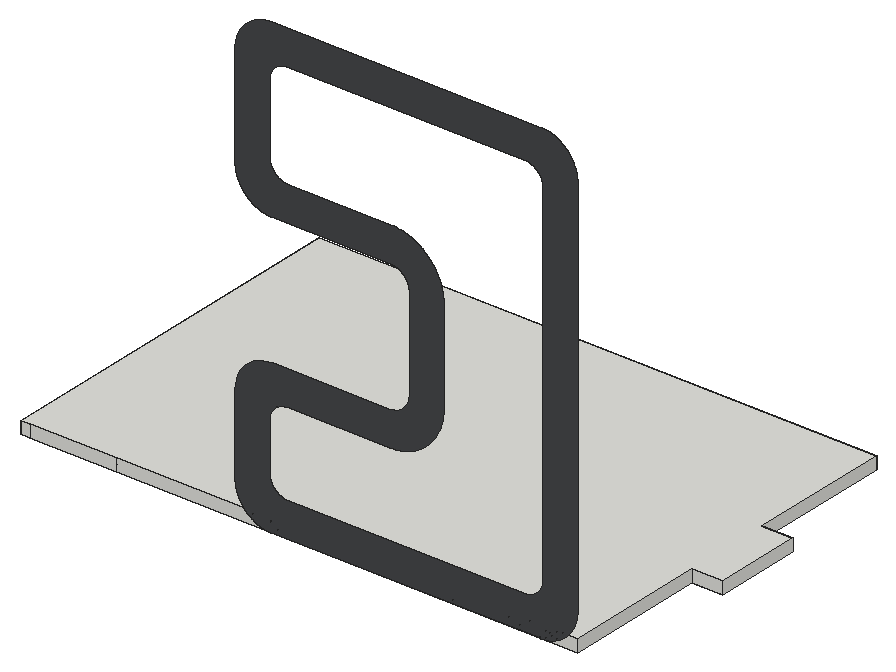
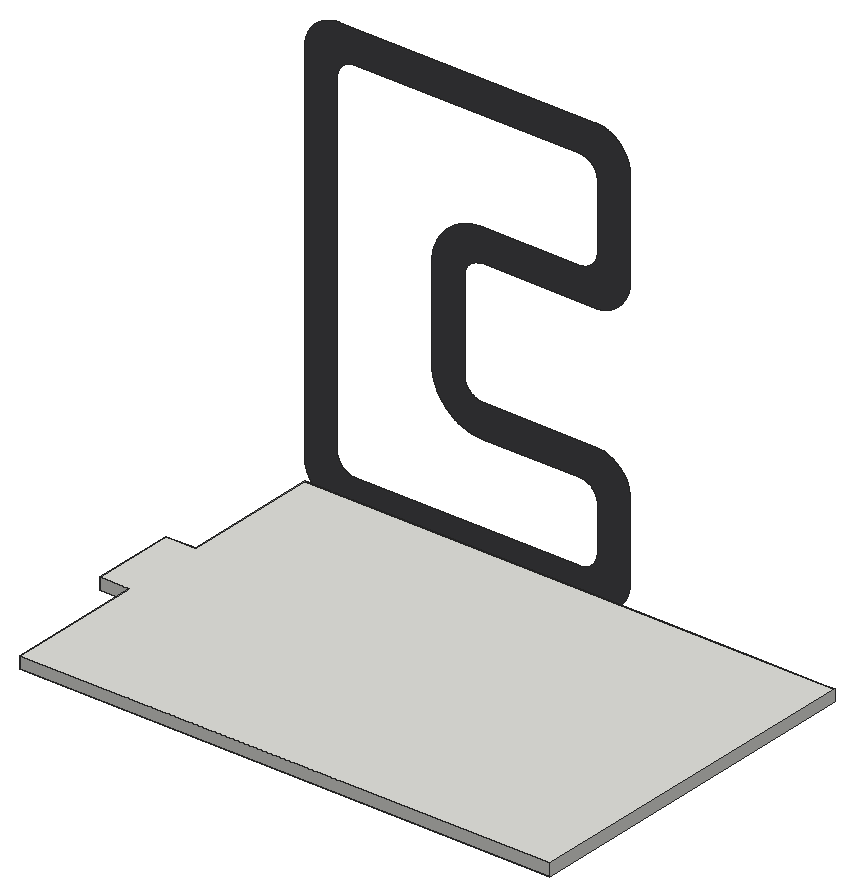
# SketchUp Ruby script. Lengths in inches.
U = 1.inch
M = Sketchup.active_model
def pt(a) = Geom::Point3d.new(a.map { |v| v * U })
def face(e, loops, mat)
  f = e.add_face(loops[0].map { |a| pt(a) })
  loops[1..].each { |l| e.add_face(l.map { |a| pt(a) }).erase! }
  f.material = f.back_material = mat if mat
  f
end
# faces: each face lists its corners as indices into pts; further lists are holes
def faces(e, pts, list, mat = nil) = list.each { |f| face(e, (f[0].is_a?(Array) ? f : [f]).map { |l| l.map { |i| pts[i] } }, mat) }
# xy, xz, yz: faces in a plane at the given z, y or x. An outline is a flat list of corners, or four numbers for a rectangle; further outlines are holes
def ring(l) = l.size == 4 ? [[l[0], l[1]], [l[2], l[1]], [l[2], l[3]], [l[0], l[3]]] : l.each_slice(2).to_a
def flat(e, list, mat, &to3) = list.each { |f| face(e, (f[0].is_a?(Array) ? f : [f]).map { |l| ring(l).map { |u, v| to3.(u, v) } }, mat) }
def xy(e, z, list, mat = nil) = flat(e, list, mat) { |x, y| [x, y, z] }
def xz(e, y, list, mat = nil) = flat(e, list, mat) { |x, z| [x, y, z] }
def yz(e, x, list, mat = nil) = flat(e, list, mat) { |y, z| [x, y, z] }
def lines(e, pts, list) = list.each { |a, b| e.add_line(pt(pts[a]), pt(pts[b])) }
# prism: a flat outline (further loops are holes) pulled along v
def prism(e, loops, v, mat = nil)
  f = face(e, loops, mat); d = Geom::Vector3d.new(v.map { |x| x * U })
  f.pushpull(f.normal.samedirection?(d) ? d.length : -d.length)
end
def box(e, o, s, mat = nil) = prism(e, [[o, [o[0] + s[0], o[1], o[2]], [o[0] + s[0], o[1] + s[1], o[2]], [o[0], o[1] + s[1], o[2]]]], [0, 0, s[2]], mat)
def at(x, y, z, deg = 0) = Geom::Transformation.translation(pt([x, y, z])) * Geom::Transformation.rotation(ORIGIN, Z_AXIS, deg.degrees)
def axes(o, x, y, z) = Geom::Transformation.new([*x, 0, *y, 0, *z, 0, *pt(o).to_a, 1])
def part(name) = M.definitions.add(name)
# library, detail: a bought-in or finely detailed component or shape, given as its bounding box
def library(name, o, s) = part(name).tap { |d| box(d.entities, o, s) }
def detail(e, o, s) = box(e.add_group.entities, o, s)
def put(e, d, t, mat = nil) = e.add_instance(d, t).tap { |i| i.material = mat if mat }
def group(e, t, mat = nil) = e.add_group.tap { |g| g.transformation = t; g.material = mat if mat }.entities
root = M.entities
M.materials.add("1432 AP 8245 TAR ROAD").color = [71, 72, 75]
xz(root,107.37,[[[278.72,155.79,278.43,155.8,278.15,155.8,277.59,155.82,277.3,155.83,277.02,155.85,276.74,155.86,276.18,155.9,275.89,155.93,275.61,155.95,274.77,156.04,274.49,156.08,274.21,156.11,273.65,156.19,273.37,156.24,273.09,156.28,272.8125,156.33,272.53,156.38,272.25,156.43,271.98,156.48,271.42,156.6,271.15,156.66,270.87,156.72,270.6,156.79,270.32,156.85,270.05,156.92,269.77,156.99,269.5,157.07,269.23,157.14,268.69,157.3,268.41,157.38,268.14,157.47,267.875,157.55,267.61,157.64,267.34,157.73,267.07,157.83,266.81,157.92,266.27,158.12,265.75,158.32,265.49,158.43,265.22,158.53,264.7,158.75,264.44,158.87,264.19,158.98,263.67,159.22,263.42,159.34,263.16,159.46,262.66,159.72,262.4,159.85,262.15,159.98,261.91,160.11,261.66,160.25,261.41,160.38,261.16,160.52,260.92,160.66,260.67,160.81,260.43,160.95,259.47,161.55,259.24,161.7,258.76,162.02,258.07,162.5,257.84,162.67,257.61,162.83,257.38,163,257.16,163.17,256.94,163.35,256.71,163.52,256.49,163.7,256.05,164.05,255.84,164.23,255.62,164.42,255.41,164.6,255.19,164.79,254.77,165.17,254.5625,165.36,254.36,165.55,254.15,165.74,253.95,165.94,253.74,166.14,253.54,166.34,253.35,166.54,252.95,166.94,252.76,167.15,252.5625,167.36,252.375,167.5625,252.18,167.77,252,167.98,251.81,168.2,251.625,168.41,251.44,168.63,251.26,168.84,251.08,169.0625,250.9,169.28,250.73,169.5,250.55,169.73,250.38,169.95,250.21,170.18,250.04,170.4,249.71,170.86,249.55,171.09,249.38,171.32,249.23,171.56,249.07,171.79,248.91,172.03,248.76,172.26,248.6,172.5,248.3,172.98,248.16,173.22,248.01,173.47,247.87,173.71,247.73,173.96,247.59,174.2,247.45,174.45,247.32,174.7,247.18,174.95,246.92,175.45,246.8,175.7,246.67,175.95,246.55,176.21,246.43,176.46,246.31,176.72,246.1875,176.98,246.07,177.24,245.96,177.49,245.85,177.75,245.74,178.02,245.63,178.28,245.53,178.54,245.42,178.8,245.32,179.07,245.23,179.33,245.13,179.6,245.03,179.86,244.76,180.67,244.68,180.9375,244.59,181.21,244.35,182.02,244.28,182.29,244.2,182.57,244.13,182.84,244.0625,183.11,243.99,183.39,243.93,183.66,243.87,183.9375,243.81,184.22,243.75,184.49,243.69,184.77,243.64,185.05,243.59,185.32,243.44,186.16,243.28,187.28,243.25,187.5625,243.22,187.84,243.1875,188.12,243.16,188.4,243.13,188.6875,243.11,188.97,243.07,189.53,243.05,189.8125,243.04,190.1,243.01,190.94,243,191.23,243,266.79,243.31,271.49,244.23,276.11,245.74,280.57,247.82,284.79,250.4375,288.71,253.54,292.25,257.08,295.35,261,297.97,265.22,300.05,269.68,301.57,274.3,302.48,279,302.79,393.24,302.79,393.47,302.8,393.71,302.81,393.94,302.82,394.18,302.83,394.41,302.85,394.65,302.87,394.88,302.89,395.12,302.92,395.58,302.98,395.82,303.01,396.28,303.09,397.2,303.29,397.89,303.47,398.11,303.53,398.34,303.6,398.5625,303.67,398.79,303.75,399.01,303.82,399.23,303.9,399.45,303.99,399.67,304.07,400.11,304.25,400.32,304.35,400.54,304.45,401.17,304.75,401.59,304.97,401.8,305.09,402,305.2,402.4,305.44,402.61,305.57,402.8,305.7,403.2,305.96,403.39,306.09,403.96,306.51,404.14,306.66,404.33,306.8,404.69,307.1,404.87,307.26,405.04,307.42,405.22,307.57,405.39,307.74,405.56,307.9,405.73,308.0625,405.89,308.23,406.06,308.4,406.22,308.57,406.375,308.75,406.53,308.92,406.6875,309.1,406.84,309.28,406.99,309.46,407.14,309.65,407.28,309.83,407.42,310.02,407.5625,310.21,407.7,310.4,407.83,310.6,407.97,310.79,408.1,310.99,408.22,311.1875,408.35,311.39,408.59,311.79,408.7,312,408.82,312.2,409.04,312.62,409.14,312.83,409.25,313.04,409.35,313.26,409.44,313.47,409.54,313.6875,409.63,313.9,409.72,314.12,409.8,314.34,409.89,314.5625,409.97,314.78,410.04,315.01,410.12,315.23,410.19,315.45,410.26,315.68,410.32,315.91,410.39,316.13,410.45,316.36,410.5,316.59,410.56,316.82,410.61,317.05,410.65,317.28,410.7,317.51,410.74,317.74,410.78,317.98,410.8125,318.21,410.85,318.44,410.875,318.68,410.9,318.91,410.92,319.15,410.96,319.61,410.98,319.85,410.99,320.09,410.99,320.32,411,320.56,411,411.03,410.99,411.26,410.99,411.5,410.98,411.73,410.96,411.97,410.94,412.2,410.92,412.4375,410.9,412.67,410.875,412.91,410.85,413.14,410.8125,413.375,410.78,413.61,410.7,414.07,410.65,414.3,410.61,414.53,410.56,414.76,410.5,414.99,410.45,415.22,410.39,415.45,410.32,415.68,410.26,415.9,410.19,416.13,410.12,416.35,410.04,416.58,409.97,416.8,409.89,417.02,409.8,417.24,409.72,417.46,409.54,417.9,409.44,418.11,409.35,418.33,409.25,418.54,409.14,418.75,409.04,418.96,408.82,419.38,408.7,419.59,408.59,419.79,408.47,420,408.35,420.2,408.22,420.4,408.1,420.6,407.97,420.79,407.83,420.99,407.7,421.18,407.5625,421.37,407.42,421.5625,407.14,421.9375,406.99,422.12,406.84,422.3,406.6875,422.48,406.53,422.66,406.375,422.84,406.22,423.01,406.06,423.18,405.89,423.35,405.73,423.52,405.56,423.69,405.22,424.01,405.04,424.17,404.87,424.33,404.33,424.78,404.14,424.93,403.96,425.07,403.39,425.49,403.2,425.625,403,425.76,402.8,425.89,402.61,426.02,402.4,426.14,401.8,426.5,401.17,426.83,400.96,426.9375,400.75,427.04,400.54,427.14,400.32,427.24,400.11,427.33,399.45,427.6,398.79,427.84,398.5625,427.91,398.34,427.98,398.11,428.05,397.89,428.12,397.43,428.24,397.2,428.29,396.97,428.35,396.51,428.45,395.82,428.57,395.58,428.61,395.12,428.67,394.88,428.69,394.65,428.72,394.41,428.74,394.18,428.75,393.94,428.77,393.71,428.78,393.47,428.79,278.72,428.79,278.43,428.8,278.15,428.8,277.59,428.82,277.3,428.83,277.02,428.85,276.74,428.86,276.18,428.9,275.89,428.93,275.61,428.95,274.77,429.04,274.49,429.08,274.21,429.11,273.65,429.19,273.37,429.24,273.09,429.28,272.8125,429.33,272.53,429.38,272.25,429.43,271.98,429.48,271.42,429.6,271.15,429.66,270.87,429.72,270.6,429.79,270.32,429.85,270.05,429.92,269.77,429.99,269.5,430.07,269.23,430.14,268.69,430.3,268.41,430.38,268.14,430.47,267.875,430.55,267.61,430.64,267.34,430.73,267.07,430.83,266.81,430.92,266.27,431.12,265.75,431.32,265.49,431.43,265.22,431.53,264.7,431.75,264.44,431.87,264.19,431.98,263.67,432.22,263.42,432.34,263.16,432.46,262.66,432.72,262.4,432.85,262.15,432.98,261.91,433.11,261.66,433.25,261.41,433.38,261.16,433.52,260.92,433.66,260.67,433.81,260.43,433.95,259.47,434.55,259.24,434.7,258.76,435.02,258.07,435.5,257.84,435.67,257.61,435.83,257.38,436,257.16,436.17,256.94,436.35,256.71,436.52,256.49,436.7,256.05,437.05,255.84,437.23,255.62,437.42,255.41,437.6,255.19,437.79,254.77,438.17,254.5625,438.36,254.36,438.55,254.15,438.74,253.95,438.94,253.74,439.14,253.54,439.34,253.35,439.54,252.95,439.94,252.76,440.15,252.5625,440.36,252.375,440.5625,252.18,440.77,252,440.98,251.81,441.2,251.625,441.41,251.44,441.63,251.26,441.84,251.08,442.0625,250.9,442.28,250.73,442.5,250.55,442.73,250.38,442.95,250.21,443.18,250.04,443.4,249.71,443.86,249.55,444.09,249.38,444.32,249.23,444.56,249.07,444.79,248.91,445.03,248.76,445.26,248.6,445.5,248.3,445.98,248.16,446.22,248.01,446.47,247.87,446.71,247.73,446.96,247.59,447.2,247.45,447.45,247.32,447.7,247.18,447.95,246.92,448.45,246.8,448.7,246.67,448.95,246.55,449.21,246.43,449.46,246.31,449.72,246.1875,449.98,246.07,450.24,245.96,450.49,245.85,450.75,245.74,451.02,245.63,451.28,245.53,451.54,245.42,451.8,245.32,452.07,245.23,452.33,245.13,452.6,245.03,452.86,244.76,453.67,244.68,453.9375,244.59,454.21,244.35,455.02,244.28,455.29,244.2,455.57,244.13,455.84,244.0625,456.11,243.99,456.39,243.93,456.66,243.87,456.9375,243.81,457.22,243.75,457.49,243.69,457.77,243.64,458.05,243.59,458.32,243.44,459.16,243.28,460.28,243.25,460.5625,243.22,460.84,243.1875,461.12,243.16,461.4,243.13,461.6875,243.11,461.97,243.07,462.53,243.05,462.8125,243.04,463.1,243.01,463.94,243,464.23,243,561.36,243.02,561.92,243.03,562.21,243.05,562.77,243.09,563.33,243.11,563.62,243.13,563.9,243.16,564.18,243.1875,564.46,243.22,564.74,243.28,565.3,243.44,566.42,243.69,567.82,243.75,568.09,243.87,568.65,243.93,568.92,243.99,569.2,244.0625,569.47,244.2,570.02,244.28,570.29,244.35,570.5625,244.43,570.84,244.59,571.38,244.68,571.65,244.76,571.92,244.85,572.19,244.94,572.45,245.03,572.72,245.13,572.99,245.23,573.25,245.32,573.52,245.42,573.78,245.53,574.04,245.63,574.31,246.07,575.35,246.1875,575.61,246.31,575.86,246.43,576.12,246.67,576.63,246.8,576.88,246.92,577.14,247.18,577.64,247.32,577.89,247.45,578.14,247.59,578.38,247.73,578.63,248.01,579.12,248.16,579.36,248.3,579.6,248.6,580.08,248.76,580.32,248.91,580.56,249.07,580.79,249.23,581.03,249.38,581.26,249.55,581.49,249.71,581.72,250.04,582.18,250.21,582.41,250.38,582.63,250.55,582.86,250.73,583.08,250.9,583.3,251.44,583.96,251.625,584.17,251.81,584.39,252,584.6,252.18,584.8125,252.375,585.02,252.5625,585.23,252.76,585.4375,252.95,585.64,253.15,585.84,253.35,586.05,253.54,586.25,253.74,586.45,253.95,586.64,254.15,586.84,254.36,587.03,254.5625,587.23,254.77,587.42,255.19,587.8,255.41,587.98,255.62,588.17,255.84,588.35,256.05,588.53,256.49,588.89,256.71,589.0625,256.94,589.24,257.38,589.58,257.84,589.92,258.07,590.08,258.3,590.25,258.76,590.57,259,590.72,259.24,590.88,259.47,591.04,259.71,591.1875,259.95,591.34,260.19,591.49,260.43,591.63,260.67,591.78,260.92,591.92,261.16,592.0625,261.41,592.2,261.66,592.34,261.91,592.47,262.15,592.61,262.4,592.74,262.66,592.87,262.91,593,263.16,593.12,263.42,593.24,263.67,593.37,263.93,593.49,264.19,593.6,264.44,593.72,265.22,594.05,265.49,594.16,265.75,594.26,266.01,594.37,266.27,594.47,266.54,594.57,266.81,594.66,267.07,594.76,267.61,594.94,268.14,595.12,268.41,595.2,268.69,595.28,269.5,595.52,269.77,595.59,270.05,595.66,270.32,595.73,270.6,595.8,270.87,595.86,271.15,595.93,271.42,595.99,271.7,596.04,271.98,596.1,272.25,596.15,272.53,596.21,272.8125,596.26,273.09,596.3,273.37,596.35,274.49,596.51,275.89,596.66,276.18,596.68,277.02,596.74,277.3,596.75,277.59,596.76,278.43,596.79,537.57,596.79,538.41,596.76,538.7,596.75,538.98,596.74,539.82,596.68,540.11,596.66,541.51,596.51,542.63,596.35,542.91,596.3,543.1875,596.26,543.47,596.21,543.75,596.15,544.02,596.1,544.3,596.04,544.58,595.99,544.85,595.93,545.13,595.86,545.4,595.8,545.68,595.73,545.95,595.66,546.23,595.59,546.5,595.52,547.31,595.28,547.59,595.2,547.86,595.12,548.39,594.94,548.93,594.76,549.19,594.66,549.46,594.57,549.73,594.47,549.99,594.37,550.25,594.26,550.51,594.16,550.78,594.05,551.56,593.72,551.81,593.6,552.07,593.49,552.33,593.37,552.58,593.24,552.84,593.12,553.09,593,553.34,592.87,553.6,592.74,553.85,592.61,554.09,592.47,554.34,592.34,554.59,592.2,554.84,592.0625,555.08,591.92,555.33,591.78,555.57,591.63,555.81,591.49,556.05,591.34,556.29,591.1875,556.53,591.04,556.76,590.88,557,590.72,557.24,590.57,557.7,590.25,557.93,590.08,558.16,589.92,558.62,589.58,559.06,589.24,559.29,589.0625,559.51,588.89,559.95,588.53,560.16,588.35,560.38,588.17,560.59,587.98,560.81,587.8,561.23,587.42,561.4375,587.23,561.64,587.03,561.85,586.84,562.05,586.64,562.26,586.45,562.46,586.25,562.65,586.05,562.85,585.84,563.05,585.64,563.24,585.4375,563.4375,585.23,563.625,585.02,563.82,584.8125,564,584.6,564.19,584.39,564.375,584.17,564.56,583.96,565.1,583.3,565.27,583.08,565.45,582.86,565.62,582.63,565.79,582.41,565.96,582.18,566.29,581.72,566.45,581.49,566.62,581.26,566.77,581.03,566.93,580.79,567.09,580.56,567.24,580.32,567.4,580.08,567.7,579.6,567.84,579.36,567.99,579.12,568.27,578.63,568.41,578.38,568.55,578.14,568.68,577.89,568.82,577.64,569.08,577.14,569.2,576.88,569.33,576.63,569.57,576.12,569.69,575.86,569.8125,575.61,569.93,575.35,570.37,574.31,570.47,574.04,570.58,573.78,570.68,573.52,570.77,573.25,570.87,572.99,570.97,572.72,571.06,572.45,571.15,572.19,571.24,571.92,571.32,571.65,571.41,571.38,571.57,570.84,571.65,570.5625,571.72,570.29,571.8,570.02,571.9375,569.47,572.01,569.2,572.07,568.92,572.13,568.65,572.25,568.09,572.31,567.82,572.56,566.42,572.72,565.3,572.78,564.74,572.8125,564.46,572.84,564.18,572.87,563.9,572.89,563.62,572.91,563.33,572.95,562.77,572.97,562.21,572.98,561.92,573,561.36,573,191.23,572.99,190.94,572.96,190.1,572.95,189.8125,572.93,189.53,572.89,188.97,572.87,188.6875,572.84,188.4,572.8125,188.12,572.78,187.84,572.75,187.5625,572.72,187.28,572.56,186.16,572.41,185.32,572.36,185.05,572.31,184.77,572.25,184.49,572.19,184.22,572.13,183.9375,572.07,183.66,572.01,183.39,571.9375,183.11,571.87,182.84,571.8,182.57,571.72,182.29,571.65,182.02,571.41,181.21,571.32,180.9375,571.24,180.67,570.97,179.86,570.87,179.6,570.77,179.33,570.68,179.07,570.58,178.8,570.47,178.54,570.37,178.28,570.26,178.02,570.15,177.75,570.04,177.49,569.93,177.24,569.8125,176.98,569.69,176.72,569.57,176.46,569.45,176.21,569.33,175.95,569.2,175.7,569.08,175.45,568.82,174.95,568.68,174.7,568.55,174.45,568.41,174.2,568.27,173.96,568.13,173.71,567.99,173.47,567.84,173.22,567.7,172.98,567.4,172.5,567.24,172.26,567.09,172.03,566.93,171.79,566.77,171.56,566.62,171.32,566.45,171.09,566.29,170.86,565.96,170.4,565.79,170.18,565.62,169.95,565.45,169.73,565.27,169.5,565.1,169.28,564.92,169.0625,564.74,168.84,564.56,168.63,564.375,168.41,564.19,168.2,564,167.98,563.82,167.77,563.625,167.5625,563.4375,167.36,563.24,167.15,563.05,166.94,562.65,166.54,562.46,166.34,562.26,166.14,562.05,165.94,561.85,165.74,561.64,165.55,561.4375,165.36,561.23,165.17,560.81,164.79,560.59,164.6,560.38,164.42,560.16,164.23,559.95,164.05,559.51,163.7,559.29,163.52,559.06,163.35,558.84,163.17,558.62,163,558.39,162.83,558.16,162.67,557.93,162.5,557.24,162.02,556.76,161.7,556.53,161.55,555.57,160.95,555.33,160.81,555.08,160.66,554.84,160.52,554.59,160.38,554.34,160.25,554.09,160.11,553.85,159.98,553.6,159.85,553.34,159.72,552.84,159.46,552.58,159.34,552.33,159.22,551.81,158.98,551.56,158.87,551.3,158.75,550.78,158.53,550.51,158.43,550.25,158.32,549.73,158.12,549.19,157.92,548.93,157.83,548.66,157.73,548.39,157.64,548.125,157.55,547.86,157.47,547.59,157.38,547.31,157.3,546.77,157.14,546.5,157.07,546.23,156.99,545.95,156.92,545.68,156.85,545.4,156.79,545.13,156.72,544.85,156.66,544.58,156.6,544.02,156.48,543.75,156.43,543.47,156.38,543.1875,156.33,542.91,156.28,542.63,156.24,542.35,156.19,541.79,156.11,541.51,156.08,541.23,156.04,540.39,155.95,540.11,155.93,539.82,155.9,539.26,155.86,538.98,155.85,538.7,155.83,538.41,155.82,537.85,155.8,537.57,155.8,537.28,155.79],[293.76,188.79,522.2,188.79,522.4,188.8,522.61,188.8,523.21,188.83,523.41,188.85,523.61,188.86,523.81,188.88,524.02,188.91,524.42,188.95,524.82,189.01,525.02,189.05,525.21,189.08,526.01,189.24,526.2,189.29,526.4,189.34,526.59,189.39,526.79,189.44,526.98,189.5,527.18,189.55,527.37,189.61,527.5625,189.67,527.75,189.74,527.95,189.8,528.14,189.87,528.32,189.94,528.51,190.01,528.7,190.09,528.89,190.16,529.07,190.24,529.26,190.32,529.44,190.4,529.63,190.49,529.81,190.57,530.17,190.75,530.35,190.85,530.53,190.94,530.71,191.04,530.88,191.14,531.06,191.24,531.4,191.44,531.58,191.55,531.92,191.77,532.08,191.88,532.25,192,532.42,192.11,532.9,192.47,533.0625,192.59,533.22,192.72,533.38,192.85,533.54,192.97,533.69,193.1,533.84,193.24,533.99,193.37,534.14,193.51,534.29,193.64,534.4375,193.78,534.58,193.92,534.73,194.0625,534.87,194.21,535.01,194.35,535.29,194.65,535.42,194.8,535.56,194.95,535.6875,195.1,535.82,195.26,535.95,195.41,536.07,195.57,536.2,195.73,536.44,196.05,536.5625,196.21,536.68,196.375,536.8,196.54,536.91,196.71,537.02,196.875,537.13,197.05,537.35,197.39,537.55,197.73,537.66,197.91,537.75,198.09,537.85,198.26,537.95,198.44,538.22,198.98,538.3,199.16,538.39,199.35,538.47,199.53,538.55,199.72,538.63,199.9,538.71,200.09,539.06,201.04,539.18,201.42,539.24,201.62,539.3,201.81,539.35,202,539.4,202.2,539.45,202.39,539.55,202.79,539.59,202.98,539.75,203.78,539.81,204.18,539.84,204.375,539.86,204.58,539.89,204.78,539.93,205.18,539.94,205.38,539.96,205.58,539.98,205.98,539.99,206.1875,540,206.39,540,546.2,539.96,547,539.94,547.2,539.93,547.41,539.89,547.81,539.86,548.01,539.84,548.21,539.75,548.81,539.71,549.01,539.67,549.2,539.55,549.8,539.5,549.99,539.4,550.39,539.35,550.58,539.3,550.78,539.12,551.35,539.06,551.55,538.78,552.31,538.71,552.49,538.55,552.87,538.47,553.05,538.39,553.24,538.3,553.42,538.22,553.6,537.95,554.14,537.75,554.5,537.66,554.68,537.55,554.85,537.45,555.02,537.35,555.2,537.02,555.71,536.8,556.04,536.68,556.21,536.5625,556.37,536.44,556.53,536.32,556.7,536.2,556.86,536.07,557.01,535.95,557.17,535.82,557.33,535.6875,557.48,535.56,557.63,535.42,557.79,535.29,557.9375,535.15,558.08,535.01,558.23,534.73,558.52,534.58,558.66,534.4375,558.8,534.29,558.94,534.14,559.08,533.99,559.21,533.84,559.35,533.54,559.61,533.22,559.87,533.0625,559.99,532.9,560.11,532.42,560.47,532.25,560.59,532.08,560.7,531.92,560.8125,531.75,560.92,531.58,561.03,531.4,561.14,531.23,561.24,531.06,561.35,530.88,561.45,530.71,561.55,530.53,561.64,530.35,561.74,529.63,562.1,529.44,562.18,529.26,562.26,529.07,562.34,528.89,562.42,528.7,562.5,528.32,562.64,528.14,562.71,527.95,562.78,527.75,562.85,527.5625,562.91,527.37,562.97,527.18,563.03,526.98,563.09,526.79,563.14,526.59,563.2,526.4,563.25,526.2,563.29,526.01,563.34,525.81,563.38,525.61,563.43,525.41,563.47,525.21,563.5,525.02,563.54,524.22,563.66,524.02,563.68,523.81,563.7,523.41,563.74,522.61,563.78,522.4,563.79,293.53,563.79,293.29,563.78,293.06,563.77,292.82,563.75,292.59,563.74,292.35,563.72,292.12,563.69,291.88,563.67,291.42,563.61,291.18,563.57,290.49,563.45,290.03,563.35,289.8,563.29,289.57,563.24,289.11,563.12,288.89,563.05,288.66,562.98,288.4375,562.91,288.21,562.84,287.55,562.6,286.89,562.33,286.68,562.24,286.46,562.14,286.25,562.04,286.04,561.9375,285.83,561.83,285.2,561.5,284.6,561.14,284.39,561.02,284.2,560.89,284,560.76,283.8,560.625,283.61,560.49,283.04,560.07,282.86,559.93,282.67,559.78,282.13,559.33,281.96,559.17,281.78,559.01,281.44,558.69,281.27,558.52,281.11,558.35,280.94,558.18,280.78,558.01,280.625,557.84,280.47,557.66,280.3125,557.48,280.16,557.3,280.01,557.12,279.86,556.9375,279.58,556.5625,279.4375,556.37,279.3,556.18,279.17,555.99,279.03,555.79,278.9,555.6,278.78,555.4,278.65,555.2,278.53,555,278.41,554.79,278.3,554.59,278.18,554.38,277.96,553.96,277.86,553.75,277.75,553.54,277.65,553.33,277.56,553.11,277.46,552.9,277.28,552.46,277.2,552.24,277.11,552.02,277.03,551.8,276.96,551.58,276.88,551.35,276.81,551.13,276.74,550.9,276.68,550.68,276.61,550.45,276.55,550.22,276.5,549.99,276.44,549.76,276.39,549.53,276.35,549.3,276.3,549.07,276.22,548.61,276.1875,548.375,276.15,548.14,276.125,547.91,276.1,547.67,276.08,547.4375,276.06,547.2,276.04,546.97,276.02,546.73,276.01,546.5,276.01,546.26,276,546.03,276,479.56,276.01,479.32,276.01,479.09,276.02,478.85,276.04,478.61,276.08,478.15,276.1,477.91,276.125,477.68,276.15,477.44,276.1875,477.21,276.22,476.98,276.26,476.74,276.3,476.51,276.35,476.28,276.39,476.05,276.44,475.82,276.5,475.59,276.55,475.36,276.61,475.13,276.68,474.91,276.74,474.68,276.81,474.45,276.88,474.23,276.96,474.01,277.03,473.78,277.11,473.5625,277.2,473.34,277.28,473.12,277.37,472.9,277.46,472.6875,277.56,472.47,277.65,472.26,277.75,472.04,277.86,471.83,277.96,471.62,278.18,471.2,278.3,471,278.41,470.79,278.65,470.39,278.78,470.1875,278.9,469.99,279.03,469.79,279.17,469.6,279.3,469.4,279.4375,469.21,279.58,469.02,279.72,468.83,279.86,468.65,280.01,468.46,280.16,468.28,280.3125,468.1,280.47,467.92,280.625,467.75,280.78,467.57,280.94,467.4,281.11,467.23,281.27,467.0625,281.44,466.9,281.61,466.74,281.78,466.57,281.96,466.42,282.13,466.26,282.31,466.1,282.67,465.8,282.86,465.66,283.04,465.51,283.61,465.09,283.8,464.96,284.2,464.7,284.39,464.57,284.6,464.44,285,464.2,285.2,464.09,285.41,463.97,285.83,463.75,286.46,463.45,286.68,463.35,286.89,463.25,287.33,463.07,287.55,462.99,287.77,462.9,287.99,462.82,288.21,462.75,288.4375,462.67,288.66,462.6,288.89,462.53,289.11,462.47,289.8,462.29,290.72,462.09,291.18,462.01,291.42,461.98,291.88,461.92,292.12,461.89,292.35,461.87,292.59,461.85,292.82,461.83,293.06,461.82,293.29,461.81,293.53,461.8,293.76,461.79,393.67,461.79,394.34,461.77,395,461.75,395.67,461.72,396.34,461.68,397,461.63,397.67,461.58,398.33,461.51,398.99,461.4375,399.66,461.36,401.64,461.06,402.29,460.9375,402.95,460.8125,403.6,460.68,404.26,460.53,404.91,460.38,405.55,460.22,406.2,460.05,406.84,459.88,407.48,459.69,408.125,459.5,408.76,459.3,409.39,459.09,410.02,458.87,410.65,458.64,411.28,458.4,411.9,458.16,412.52,457.91,413.13,457.65,414.35,457.11,414.96,456.82,415.56,456.53,416.15,456.23,416.75,455.93,417.34,455.61,417.92,455.29,418.5,454.96,419.08,454.62,419.65,454.28,420.21,453.92,420.78,453.5625,421.33,453.2,421.89,452.82,422.43,452.44,422.98,452.05,423.51,451.66,424.05,451.25,424.57,450.84,425.1,450.43,426.12,449.57,426.625,449.14,427.125,448.69,427.62,448.24,428.11,447.79,428.59,447.32,429.0625,446.85,429.53,446.38,429.99,445.9,430.45,445.41,430.9,444.92,431.34,444.42,431.78,443.91,432.21,443.4,432.63,442.89,433.05,442.37,433.46,441.84,433.86,441.31,434.26,440.77,434.65,440.23,435.03,439.68,435.77,438.57,436.13,438.01,436.48,437.4375,436.83,436.87,437.17,436.29,437.5,435.71,437.82,435.13,438.44,433.95,438.74,433.35,439.03,432.75,439.32,432.14,439.59,431.54,439.86,430.92,440.12,430.31,440.37,429.69,440.61,429.07,440.85,428.44,441.07,427.82,441.29,427.19,441.5,426.55,441.71,425.92,442.09,424.64,442.26,423.99,442.43,423.35,442.59,422.7,442.89,421.4,443.02,420.74,443.15,420.09,443.37,418.77,443.47,418.11,443.5625,417.45,443.65,416.79,443.79,415.46,443.84,414.79,443.89,414.13,443.93,413.46,443.96,412.79,443.98,412.13,444,411.46,444,320.125,443.98,319.46,443.96,318.79,443.93,318.12,443.89,317.46,443.84,316.79,443.79,316.125,443.72,315.46,443.65,314.8,443.5625,314.14,443.47,313.47,443.37,312.8125,443.26,312.16,443.15,311.5,443.02,310.84,442.89,310.1875,442.74,309.54,442.59,308.89,442.43,308.24,442.26,307.59,442.09,306.95,441.71,305.67,441.5,305.03,441.29,304.4,440.85,303.14,440.61,302.52,440.37,301.89,440.12,301.28,439.86,300.66,439.32,299.44,438.74,298.24,438.44,297.64,437.82,296.46,437.5,295.87,437.17,295.29,436.83,294.72,436.48,294.14,436.13,293.58,435.77,293.02,435.4,292.46,435.03,291.91,434.65,291.36,434.26,290.82,433.86,290.28,433.46,289.75,433.05,289.22,432.21,288.18,431.78,287.67,430.9,286.67,430.45,286.17,429.99,285.6875,429.53,285.2,429.0625,284.73,428.59,284.26,428.11,283.8,427.62,283.34,427.125,282.89,426.625,282.45,426.12,282.01,425.61,281.58,425.1,281.16,424.57,280.74,424.05,280.33,423.51,279.93,422.98,279.53,422.43,279.14,421.89,278.76,421.33,278.39,420.78,278.02,420.21,277.66,419.65,277.31,419.08,276.96,417.92,276.29,417.34,275.97,416.75,275.66,416.15,275.35,415.56,275.05,414.96,274.76,413.74,274.2,413.13,273.93,412.52,273.67,411.9,273.42,411.28,273.18,410.65,272.94,409.39,272.5,408.76,272.29,408.125,272.09,407.48,271.89,406.2,271.53,405.55,271.36,404.91,271.2,404.26,271.05,403.6,270.91,402.95,270.77,402.29,270.65,401.64,270.53,400.98,270.42,400.32,270.32,399.66,270.23,398.99,270.15,398.33,270.07,397.67,270.01,397,269.95,396.34,269.9,395.67,269.86,395,269.83,394.34,269.81,393,269.79,293.58,269.79,292.74,269.75,292.32,269.71,292.12,269.69,291.91,269.67,291.7,269.64,291.49,269.62,291.28,269.59,291.08,269.55,290.87,269.52,290.66,269.48,290.46,269.44,290.25,269.4,290.05,269.35,289.84,269.31,289.64,269.26,289.4375,269.2,289.23,269.15,288.43,268.91,288.03,268.77,287.84,268.7,287.44,268.56,287.06,268.4,286.86,268.32,286.67,268.23,286.48,268.15,286.1,267.97,285.91,267.87,285.73,267.78,285.54,267.68,285.36,267.58,285.17,267.48,284.81,267.27,284.45,267.05,284.27,266.9375,284.12,266.79,282,266.79,282,265.16,281.83,265.05,281.53,264.77,281.39,264.63,281.24,264.49,281.1,264.35,280.96,264.2,280.83,264.06,280.6875,263.91,280.55,263.76,280.29,263.46,280.16,263.3,280.03,263.15,279.91,262.99,279.78,262.83,279.42,262.35,279.3,262.18,279.1875,262.02,279.07,261.85,278.96,261.68,278.85,261.52,278.74,261.35,278.64,261.17,278.53,261,278.43,260.83,278.33,260.65,278.23,260.48,278.14,260.3,278.04,260.12,277.77,259.58,277.6875,259.4,277.6,259.22,277.52,259.03,277.44,258.85,277.36,258.66,277.29,258.48,277.21,258.29,277,257.72,276.875,257.34,276.82,257.15,276.76,256.96,276.7,256.76,276.65,256.57,276.59,256.375,276.54,256.18,276.49,255.98,276.45,255.79,276.41,255.59,276.36,255.39,276.32,255.2,276.29,255,276.25,254.8,276.16,254.2,276.14,254,276.11,253.8,276.07,253.4,276.06,253.2,276.04,253,276.01,252.4,276,252.19,276,206.56,276.01,206.32,276.01,206.09,276.02,205.85,276.04,205.61,276.08,205.15,276.1,204.91,276.125,204.68,276.15,204.44,276.1875,204.21,276.22,203.98,276.26,203.74,276.3,203.51,276.35,203.28,276.39,203.05,276.44,202.82,276.5,202.59,276.55,202.36,276.61,202.13,276.68,201.91,276.74,201.68,276.81,201.45,276.88,201.23,276.96,201.01,277.03,200.78,277.11,200.5625,277.2,200.34,277.28,200.12,277.37,199.9,277.46,199.6875,277.56,199.47,277.65,199.26,277.75,199.04,277.86,198.83,277.96,198.62,278.18,198.2,278.3,198,278.41,197.79,278.65,197.39,278.78,197.1875,278.9,196.99,279.03,196.79,279.17,196.6,279.3,196.4,279.4375,196.21,279.58,196.02,279.72,195.83,279.86,195.65,280.01,195.46,280.16,195.28,280.3125,195.1,280.47,194.92,280.625,194.75,280.78,194.57,280.94,194.4,281.11,194.23,281.27,194.0625,281.44,193.9,281.61,193.74,281.78,193.57,281.96,193.42,282.13,193.26,282.31,193.1,282.67,192.8,282.86,192.66,283.04,192.51,283.61,192.09,283.8,191.96,284.2,191.7,284.39,191.57,284.6,191.44,285,191.2,285.2,191.09,285.41,190.97,285.83,190.75,286.46,190.45,286.68,190.35,286.89,190.25,287.33,190.07,287.55,189.99,287.77,189.9,287.99,189.82,288.21,189.75,288.4375,189.67,288.66,189.6,288.89,189.53,289.11,189.47,289.8,189.29,290.72,189.09,291.18,189.01,291.42,188.98,291.88,188.92,292.12,188.89,292.35,188.87,292.59,188.85,292.82,188.83,293.06,188.82,293.29,188.81,293.53,188.8]]],"1432 AP 8245 TAR ROAD")
g1 = group(root,at(45,116.37,155.79))
prism(g1,[[[-9,-9,0],[-9,351,0],[528,351,0],[528,213,0],[558,213,0],[558,129,0],[528,129,0],[528,-9,0],[84,-9,0],[0,-9,0]]],[0,0,12])
